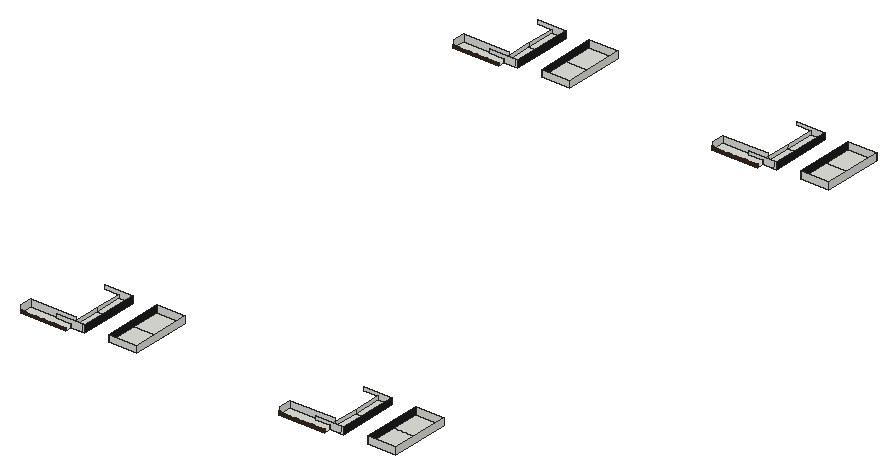
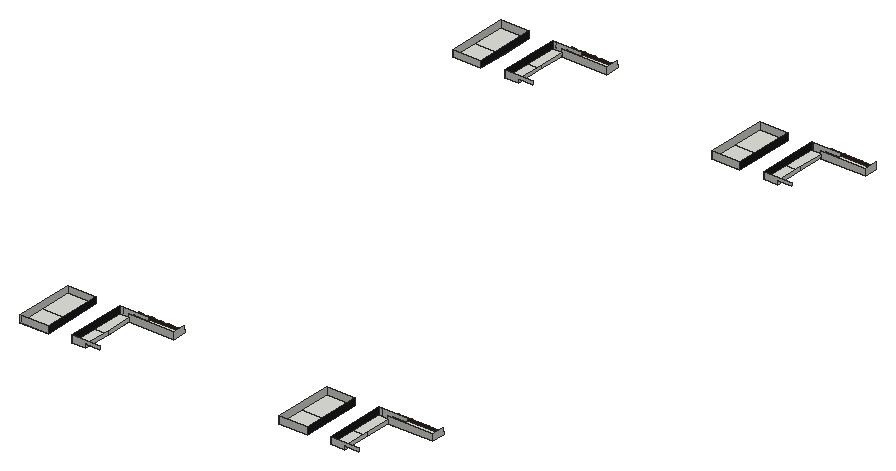
# SketchUp Ruby script. Lengths in inches.
U = 1.inch
M = Sketchup.active_model
def pt(a) = Geom::Point3d.new(a.map { |v| v * U })
def face(e, loops, mat)
  f = e.add_face(loops[0].map { |a| pt(a) })
  loops[1..].each { |l| e.add_face(l.map { |a| pt(a) }).erase! }
  f.material = f.back_material = mat if mat
  f
end
# faces: each face lists its corners as indices into pts; further lists are holes
def faces(e, pts, list, mat = nil) = list.each { |f| face(e, (f[0].is_a?(Array) ? f : [f]).map { |l| l.map { |i| pts[i] } }, mat) }
# xy, xz, yz: faces in a plane at the given z, y or x. An outline is a flat list of corners, or four numbers for a rectangle; further outlines are holes
def ring(l) = l.size == 4 ? [[l[0], l[1]], [l[2], l[1]], [l[2], l[3]], [l[0], l[3]]] : l.each_slice(2).to_a
def flat(e, list, mat, &to3) = list.each { |f| face(e, (f[0].is_a?(Array) ? f : [f]).map { |l| ring(l).map { |u, v| to3.(u, v) } }, mat) }
def xy(e, z, list, mat = nil) = flat(e, list, mat) { |x, y| [x, y, z] }
def xz(e, y, list, mat = nil) = flat(e, list, mat) { |x, z| [x, y, z] }
def yz(e, x, list, mat = nil) = flat(e, list, mat) { |y, z| [x, y, z] }
def lines(e, pts, list) = list.each { |a, b| e.add_line(pt(pts[a]), pt(pts[b])) }
# prism: a flat outline (further loops are holes) pulled along v
def prism(e, loops, v, mat = nil)
  f = face(e, loops, mat); d = Geom::Vector3d.new(v.map { |x| x * U })
  f.pushpull(f.normal.samedirection?(d) ? d.length : -d.length)
end
def box(e, o, s, mat = nil) = prism(e, [[o, [o[0] + s[0], o[1], o[2]], [o[0] + s[0], o[1] + s[1], o[2]], [o[0], o[1] + s[1], o[2]]]], [0, 0, s[2]], mat)
def at(x, y, z, deg = 0) = Geom::Transformation.translation(pt([x, y, z])) * Geom::Transformation.rotation(ORIGIN, Z_AXIS, deg.degrees)
def axes(o, x, y, z) = Geom::Transformation.new([*x, 0, *y, 0, *z, 0, *pt(o).to_a, 1])
def part(name) = M.definitions.add(name)
# library, detail: a bought-in or finely detailed component or shape, given as its bounding box
def library(name, o, s) = part(name).tap { |d| box(d.entities, o, s) }
def detail(e, o, s) = box(e.add_group.entities, o, s)
def put(e, d, t, mat = nil) = e.add_instance(d, t).tap { |i| i.material = mat if mat }
def group(e, t, mat = nil) = e.add_group.tap { |g| g.transformation = t; g.material = mat if mat }.entities
root = M.entities
M.materials.add("[Color M08]").color = [30, 30, 30]
M.materials.add("[Wood Veneer 01]").color = [66, 38, 20]
xy(root,230.89,[[2010.28,566.68,2164.35,611.02],[2889.03,566.68,3043.1,611.02],[2010.28,2402.3,2164.35,2446.65],[2889.03,2402.3,3043.1,2446.65]])
xy(root,231,[[2164.35,589.83,2211.2,697.21],[2291.96,589.83,2387.27,697.21],[3043.1,589.83,3089.95,697.21],[3170.71,589.83,3266.02,697.21],[2164.35,697.21,2211.2,792.52],
  [2291.96,697.21,2387.27,792.52],[3043.1,697.21,3089.95,792.52],[3170.71,697.21,3266.02,792.52],[2164.35,2425.46,2211.2,2532.83],[2291.96,2425.46,2387.27,2532.83],
  [3043.1,2425.46,3089.95,2532.83],[3170.71,2425.46,3266.02,2532.83],[2164.35,2532.83,2211.2,2628.15],[2291.96,2532.83,2387.27,2628.15],[3043.1,2532.83,3089.95,2628.15],
  [3170.71,2532.83,3266.02,2628.15]])
xz(root,566.68,[[2010.28,230.89,2164.35,230.89,2164.35,240.89,2162.52,240.1,2161.96,239.96,2161.4375,239.81,2160.75,239.53,2160.2,239.49,2159.48,239.42,2158.68,239.28,2157.91,239.15,2157.28,238.9,2155.89,238.9,2155.13,238.89,2154.45,238.89,2153.77,238.88,2153.23,238.875,2152.47,238.86,2151.73,238.83,2151.16,238.8,2150.58,238.74,2149.92,238.6,2149.35,238.51,2148.82,238.33,2148.13,238.08,2147.45,237.84,2146.76,237.5625,2146.16,237.47,2145.48,237.4,2144.75,237.42,2144.18,237.45,2143.59,237.51,2142.99,237.59,2142.45,237.71,2141.62,238,2140.91,238.33,2140.36,238.57,2139.86,238.86,2139.34,238.96,2138.65,239.02,2137.97,239.125,2137.23,239.04,2136.66,238.66,2136.07,238.61,2135.41,238.55,2134.89,238.27,2134.21,238.18,2133.53,238.18,2132.86,238.11,2132.33,238.15,2131.51,238.19,2130.9375,238.26,2130.37,238.48,2129.71,238.56,2129.14,238.67,2128.62,239.01,2127.9375,239.18,2127.3125,239.5,2126.55,239.65,2125.9375,239.8,2125.18,239.96,2124.53,240.23,2123.95,240.27,2123.3,240.43,2122.73,240.43,2122.15,240.42,2121.625,240.41,2120.93,240.4,2120.24,240.37,2119.55,240.33,2118.87,240.27,2118.19,240.17,2117.57,239.97,2116.92,239.75,2116.18,239.375,2115.39,239.08,2114.51,238.72,2113.76,238.46,2112.54,238.14,2111.42,237.88,2110.77,237.87,2109.9,237.74,2109.19,237.79,2108.42,237.86,2107.79,238.15,2107.02,238.19,2106.4,238.25,2105.64,238.45,2104.95,238.62,2100.06,238.62,2099.5,238.625,2098.64,238.625,2097.95,238.63,2097.33,238.64,2096.55,238.65,2095.88,238.66,2095.19,238.6875,2094.52,238.73,2094.04,238.78,2093.16,238.93,2092.39,239.07,2091.84,239.16,2090.99,239.44,2090.32,239.56,2089.71,239.72,2088.98,239.7,2088.42,239.69,2087.83,239.65,2087.21,239.6,2086.72,239.54,2085.91,239.31,2084.91,239.22,2084.33,239.12,2083.6875,238.76,2083.05,238.51,2082.49,238.375,2082.05,238.02,2081.35,237.74,2080.73,237.43,2079.88,237.22,2079.2,236.98,2078.59,237.01,2077.9,237.04,2077.14,237.11,2076.45,237.2,2075.92,237.33,2075.25,237.68,2074.3125,237.96,2073.75,238.28,2072.97,238.43,2072.19,238.78,2071.52,238.79,2070.98,238.8,2070.22,238.83,2069.47,238.875,2068.9,238.94,2068.32,239.04,2067.66,239.29,2067.08,239.53,2066.55,239.7,2065.86,239.92,2065.23,240.11,2064.45,240.27,2063.83,240.25,2063.125,240.23,2062.36,240.19,2061.6875,240.12,2061.03,240.03,2060.39,239.85,2059.84,239.52,2059.28,239.35,2058.69,239.18,2058.18,238.86,2057.49,238.72,2056.67,238.59,2056.16,238.34,2050.59,238.34,2049.91,238.33,2048.68,238.33,2047.96,238.32,2047.11,238.3,2046.48,238.28,2045.73,238.26,2045.1,238.15,2044.34,238.13,2043.79,238.1,2042.9375,237.98,2042.32,237.94,2041.56,237.89,2040.89,237.65,2039.58,237.65,2038.89,237.66,2038.14,237.67,2037.54,237.68,2036.93,237.71,2036.22,237.76,2035.53,237.82,2034.87,237.9,2033.93,238.21,2033.46,238.31,2032.55,238.43,2031.9,238.74,2031.32,239.11,2030.74,239.38,2030.28,239.71,2029.58,240.11,2028.89,240.09,2028.23,240.05,2027.64,239.99,2026.91,239.88,2026.36,239.69,2025.78,239.55,2025.22,238.9375,2024.69,238.77,2023.95,238.79,2023.08,238.8,2022.57,238.82,2021.53,238.92,2020.84,238.93,2020.14,238.94,2019.44,238.97,2018.76,239.03,2018.07,239.09,2017.29,239.19,2016.78,239.52,2016.22,239.64,2015.77,239.86,2014.98,240.2,2014.38,240.59,2013.84,240.85,2012.82,241.55,2011.55,241.69,2010.34,241.52,2010.28,241.52],[2889.03,230.89,3043.1,230.89,3043.1,240.89,3041.27,240.1,3040.71,239.96,3040.1875,239.81,3039.5,239.53,3038.95,239.49,3038.23,239.42,3037.43,239.28,3036.66,239.15,3036.03,238.9,3034.64,238.9,3033.88,238.89,3033.2,238.89,3032.52,238.88,3031.98,238.875,3031.22,238.86,3030.48,238.83,3029.91,238.8,3029.33,238.74,3028.67,238.6,3028.1,238.51,3027.57,238.33,3026.88,238.08,3026.2,237.84,3025.51,237.5625,3024.91,237.47,3024.23,237.4,3023.5,237.42,3022.93,237.45,3022.34,237.51,3021.74,237.59,3021.2,237.71,3020.37,238,3019.66,238.33,3019.11,238.57,3018.61,238.86,3018.09,238.96,3017.4,239.02,3016.72,239.125,3015.98,239.04,3015.41,238.66,3014.82,238.61,3014.16,238.55,3013.64,238.27,3012.96,238.18,3012.28,238.18,3011.61,238.11,3011.08,238.15,3010.26,238.19,3009.6875,238.26,3009.12,238.48,3008.46,238.56,3007.89,238.67,3007.37,239.01,3006.6875,239.18,3006.0625,239.5,3005.3,239.65,3004.6875,239.8,3003.93,239.96,3003.28,240.23,3002.7,240.27,3002.05,240.43,3001.48,240.43,3000.9,240.42,3000.375,240.41,2999.68,240.4,2998.99,240.37,2998.3,240.33,2997.62,240.27,2996.94,240.17,2996.32,239.97,2995.67,239.75,2994.93,239.375,2994.14,239.08,2993.26,238.72,2992.51,238.46,2991.29,238.14,2990.17,237.88,2989.52,237.87,2988.65,237.74,2987.94,237.79,2987.17,237.86,2986.54,238.15,2985.77,238.19,2985.15,238.25,2984.39,238.45,2983.7,238.62,2978.81,238.62,2978.25,238.625,2977.39,238.625,2976.7,238.63,2976.08,238.64,2975.3,238.65,2974.63,238.66,2973.94,238.6875,2973.27,238.73,2972.79,238.78,2971.91,238.93,2971.14,239.07,2970.59,239.16,2969.74,239.44,2969.07,239.56,2968.46,239.72,2967.73,239.7,2967.17,239.69,2966.58,239.65,2965.96,239.6,2965.47,239.54,2964.66,239.31,2963.66,239.22,2963.08,239.12,2962.4375,238.76,2961.8,238.51,2961.24,238.375,2960.8,238.02,2960.1,237.74,2959.48,237.43,2958.63,237.22,2957.95,236.98,2957.34,237.01,2956.65,237.04,2955.89,237.11,2955.2,237.2,2954.67,237.33,2954,237.68,2953.0625,237.96,2952.5,238.28,2951.72,238.43,2950.94,238.78,2950.27,238.79,2949.73,238.8,2948.97,238.83,2948.22,238.875,2947.65,238.94,2947.07,239.04,2946.41,239.29,2945.83,239.53,2945.3,239.7,2944.61,239.92,2943.98,240.11,2943.2,240.27,2942.58,240.25,2941.875,240.23,2941.11,240.19,2940.4375,240.12,2939.78,240.03,2939.14,239.85,2938.59,239.52,2938.03,239.35,2937.44,239.18,2936.93,238.86,2936.24,238.72,2935.42,238.59,2934.91,238.34,2929.34,238.34,2928.66,238.33,2927.43,238.33,2926.71,238.32,2925.86,238.3,2925.23,238.28,2924.48,238.26,2923.85,238.15,2923.09,238.13,2922.54,238.1,2921.6875,237.98,2921.07,237.94,2920.31,237.89,2919.64,237.65,2918.33,237.65,2917.64,237.66,2916.89,237.67,2916.29,237.68,2915.68,237.71,2914.97,237.76,2914.28,237.82,2913.62,237.9,2912.68,238.21,2912.21,238.31,2911.3,238.43,2910.65,238.74,2910.07,239.11,2909.49,239.38,2909.03,239.71,2908.33,240.11,2907.64,240.09,2906.98,240.05,2906.39,239.99,2905.66,239.88,2905.11,239.69,2904.53,239.55,2903.97,238.9375,2903.44,238.77,2902.7,238.79,2901.83,238.8,2901.32,238.82,2900.28,238.92,2899.59,238.93,2898.89,238.94,2898.19,238.97,2897.51,239.03,2896.82,239.09,2896.04,239.19,2895.53,239.52,2894.97,239.64,2894.52,239.86,2893.73,240.2,2893.13,240.59,2892.59,240.85,2891.57,241.55,2890.3,241.69,2889.09,241.52,2889.03,241.52]],"[Wood Veneer 01]")
xz(root,589.83,[[2164.35,231,2202.28,231,2202.28,254.5,2115.89,254.5,2115.89,242.625,2164.35,242.625],[2202.28,231,2211.2,254.5],[2291.96,231,2387.27,254.5],[3043.1,231,3081.03,231,3081.03,254.5,2994.64,254.5,2994.64,242.625,3043.1,242.625],[3081.03,231,3089.95,254.5],
  [3170.71,231,3266.02,254.5]])
xz(root,611.02,[[2010.28,230.89,2164.35,254.5],[2889.03,230.89,3043.1,254.5]])
xz(root,792.52,[[2164.35,231,2164.35,242.625,2115.89,242.625,2115.89,254.5,2211.2,254.5,2211.2,231],[2291.96,231,2387.27,254.5],[3043.1,231,3043.1,242.625,2994.64,242.625,2994.64,254.5,3089.95,254.5,3089.95,231],[3170.71,231,3266.02,254.5]])
xz(root,2402.3,[[2010.28,230.89,2164.35,230.89,2164.35,240.89,2162.52,240.1,2161.96,239.96,2161.4375,239.81,2160.75,239.53,2160.2,239.49,2159.48,239.42,2158.68,239.28,2157.91,239.15,2157.28,238.9,2155.89,238.9,2155.13,238.89,2154.45,238.89,2153.77,238.88,2153.23,238.875,2152.47,238.86,2151.73,238.83,2151.16,238.8,2150.58,238.74,2149.92,238.6,2149.35,238.51,2148.82,238.33,2148.13,238.08,2147.45,237.84,2146.76,237.5625,2146.16,237.47,2145.48,237.4,2144.75,237.42,2144.18,237.45,2143.59,237.51,2142.99,237.59,2142.45,237.71,2141.62,238,2140.91,238.33,2140.36,238.57,2139.86,238.86,2139.34,238.96,2138.65,239.02,2137.97,239.125,2137.23,239.04,2136.66,238.66,2136.07,238.61,2135.41,238.55,2134.89,238.27,2134.21,238.18,2133.53,238.18,2132.86,238.11,2132.33,238.15,2131.51,238.19,2130.9375,238.26,2130.37,238.48,2129.71,238.56,2129.14,238.67,2128.62,239.01,2127.9375,239.18,2127.3125,239.5,2126.55,239.65,2125.9375,239.8,2125.18,239.96,2124.53,240.23,2123.95,240.27,2123.3,240.43,2122.73,240.43,2122.15,240.42,2121.625,240.41,2120.93,240.4,2120.24,240.37,2119.55,240.33,2118.87,240.27,2118.19,240.17,2117.57,239.97,2116.92,239.75,2116.18,239.375,2115.39,239.08,2114.51,238.72,2113.76,238.46,2112.54,238.14,2111.42,237.88,2110.77,237.87,2109.9,237.74,2109.19,237.79,2108.42,237.86,2107.79,238.15,2107.02,238.19,2106.4,238.25,2105.64,238.45,2104.95,238.62,2100.06,238.62,2099.5,238.625,2098.64,238.625,2097.95,238.63,2097.33,238.64,2096.55,238.65,2095.88,238.66,2095.19,238.6875,2094.52,238.73,2094.04,238.78,2093.16,238.93,2092.39,239.07,2091.84,239.16,2090.99,239.44,2090.32,239.56,2089.71,239.72,2088.98,239.7,2088.42,239.69,2087.83,239.65,2087.21,239.6,2086.72,239.54,2085.91,239.31,2084.91,239.22,2084.33,239.12,2083.6875,238.76,2083.05,238.51,2082.49,238.375,2082.05,238.02,2081.35,237.74,2080.73,237.43,2079.88,237.22,2079.2,236.98,2078.59,237.01,2077.9,237.04,2077.14,237.11,2076.45,237.2,2075.92,237.33,2075.25,237.68,2074.3125,237.96,2073.75,238.28,2072.97,238.43,2072.19,238.78,2071.52,238.79,2070.98,238.8,2070.22,238.83,2069.47,238.875,2068.9,238.94,2068.32,239.04,2067.66,239.29,2067.08,239.53,2066.55,239.7,2065.86,239.92,2065.23,240.11,2064.45,240.27,2063.83,240.25,2063.125,240.23,2062.36,240.19,2061.6875,240.12,2061.03,240.03,2060.39,239.85,2059.84,239.52,2059.28,239.35,2058.69,239.18,2058.18,238.86,2057.49,238.72,2056.67,238.59,2056.16,238.34,2050.59,238.34,2049.91,238.33,2048.68,238.33,2047.96,238.32,2047.11,238.3,2046.48,238.28,2045.73,238.26,2045.1,238.15,2044.34,238.13,2043.79,238.1,2042.9375,237.98,2042.32,237.94,2041.56,237.89,2040.89,237.65,2039.58,237.65,2038.89,237.66,2038.14,237.67,2037.54,237.68,2036.93,237.71,2036.22,237.76,2035.53,237.82,2034.87,237.9,2033.93,238.21,2033.46,238.31,2032.55,238.43,2031.9,238.74,2031.32,239.11,2030.74,239.38,2030.28,239.71,2029.58,240.11,2028.89,240.09,2028.23,240.05,2027.64,239.99,2026.91,239.88,2026.36,239.69,2025.78,239.55,2025.22,238.9375,2024.69,238.77,2023.95,238.79,2023.08,238.8,2022.57,238.82,2021.53,238.92,2020.84,238.93,2020.14,238.94,2019.44,238.97,2018.76,239.03,2018.07,239.09,2017.29,239.19,2016.78,239.52,2016.22,239.64,2015.77,239.86,2014.98,240.2,2014.38,240.59,2013.84,240.85,2012.82,241.55,2011.55,241.69,2010.34,241.52,2010.28,241.52],[2889.03,230.89,3043.1,230.89,3043.1,240.89,3041.27,240.1,3040.71,239.96,3040.1875,239.81,3039.5,239.53,3038.95,239.49,3038.23,239.42,3037.43,239.28,3036.66,239.15,3036.03,238.9,3034.64,238.9,3033.88,238.89,3033.2,238.89,3032.52,238.88,3031.98,238.875,3031.22,238.86,3030.48,238.83,3029.91,238.8,3029.33,238.74,3028.67,238.6,3028.1,238.51,3027.57,238.33,3026.88,238.08,3026.2,237.84,3025.51,237.5625,3024.91,237.47,3024.23,237.4,3023.5,237.42,3022.93,237.45,3022.34,237.51,3021.74,237.59,3021.2,237.71,3020.37,238,3019.66,238.33,3019.11,238.57,3018.61,238.86,3018.09,238.96,3017.4,239.02,3016.72,239.125,3015.98,239.04,3015.41,238.66,3014.82,238.61,3014.16,238.55,3013.64,238.27,3012.96,238.18,3012.28,238.18,3011.61,238.11,3011.08,238.15,3010.26,238.19,3009.6875,238.26,3009.12,238.48,3008.46,238.56,3007.89,238.67,3007.37,239.01,3006.6875,239.18,3006.0625,239.5,3005.3,239.65,3004.6875,239.8,3003.93,239.96,3003.28,240.23,3002.7,240.27,3002.05,240.43,3001.48,240.43,3000.9,240.42,3000.375,240.41,2999.68,240.4,2998.99,240.37,2998.3,240.33,2997.62,240.27,2996.94,240.17,2996.32,239.97,2995.67,239.75,2994.93,239.375,2994.14,239.08,2993.26,238.72,2992.51,238.46,2991.29,238.14,2990.17,237.88,2989.52,237.87,2988.65,237.74,2987.94,237.79,2987.17,237.86,2986.54,238.15,2985.77,238.19,2985.15,238.25,2984.39,238.45,2983.7,238.62,2978.81,238.62,2978.25,238.625,2977.39,238.625,2976.7,238.63,2976.08,238.64,2975.3,238.65,2974.63,238.66,2973.94,238.6875,2973.27,238.73,2972.79,238.78,2971.91,238.93,2971.14,239.07,2970.59,239.16,2969.74,239.44,2969.07,239.56,2968.46,239.72,2967.73,239.7,2967.17,239.69,2966.58,239.65,2965.96,239.6,2965.47,239.54,2964.66,239.31,2963.66,239.22,2963.08,239.12,2962.4375,238.76,2961.8,238.51,2961.24,238.375,2960.8,238.02,2960.1,237.74,2959.48,237.43,2958.63,237.22,2957.95,236.98,2957.34,237.01,2956.65,237.04,2955.89,237.11,2955.2,237.2,2954.67,237.33,2954,237.68,2953.0625,237.96,2952.5,238.28,2951.72,238.43,2950.94,238.78,2950.27,238.79,2949.73,238.8,2948.97,238.83,2948.22,238.875,2947.65,238.94,2947.07,239.04,2946.41,239.29,2945.83,239.53,2945.3,239.7,2944.61,239.92,2943.98,240.11,2943.2,240.27,2942.58,240.25,2941.875,240.23,2941.11,240.19,2940.4375,240.12,2939.78,240.03,2939.14,239.85,2938.59,239.52,2938.03,239.35,2937.44,239.18,2936.93,238.86,2936.24,238.72,2935.42,238.59,2934.91,238.34,2929.34,238.34,2928.66,238.33,2927.43,238.33,2926.71,238.32,2925.86,238.3,2925.23,238.28,2924.48,238.26,2923.85,238.15,2923.09,238.13,2922.54,238.1,2921.6875,237.98,2921.07,237.94,2920.31,237.89,2919.64,237.65,2918.33,237.65,2917.64,237.66,2916.89,237.67,2916.29,237.68,2915.68,237.71,2914.97,237.76,2914.28,237.82,2913.62,237.9,2912.68,238.21,2912.21,238.31,2911.3,238.43,2910.65,238.74,2910.07,239.11,2909.49,239.38,2909.03,239.71,2908.33,240.11,2907.64,240.09,2906.98,240.05,2906.39,239.99,2905.66,239.88,2905.11,239.69,2904.53,239.55,2903.97,238.9375,2903.44,238.77,2902.7,238.79,2901.83,238.8,2901.32,238.82,2900.28,238.92,2899.59,238.93,2898.89,238.94,2898.19,238.97,2897.51,239.03,2896.82,239.09,2896.04,239.19,2895.53,239.52,2894.97,239.64,2894.52,239.86,2893.73,240.2,2893.13,240.59,2892.59,240.85,2891.57,241.55,2890.3,241.69,2889.09,241.52,2889.03,241.52]],"[Wood Veneer 01]")
xz(root,2425.46,[[2164.35,231,2202.28,231,2202.28,254.5,2115.89,254.5,2115.89,242.625,2164.35,242.625],[2202.28,231,2211.2,254.5],[2291.96,231,2387.27,254.5],[3043.1,231,3081.03,231,3081.03,254.5,2994.64,254.5,2994.64,242.625,3043.1,242.625],[3081.03,231,3089.95,254.5],
  [3170.71,231,3266.02,254.5]])
xz(root,2446.65,[[2010.28,230.89,2164.35,254.5],[2889.03,230.89,3043.1,254.5]])
xz(root,2628.15,[[2164.35,231,2164.35,242.625,2115.89,242.625,2115.89,254.5,2211.2,254.5,2211.2,231],[2291.96,231,2387.27,254.5],[3043.1,231,3043.1,242.625,2994.64,242.625,2994.64,254.5,3089.95,254.5,3089.95,231],[3170.71,231,3266.02,254.5]])
yz(root,2010.28,[[566.68,230.89,566.68,241.52,568.68,241.52,568.68,254.5,611.02,254.5,611.02,230.89],[2402.3,230.89,2402.3,241.52,2404.3,241.52,2404.3,254.5,2446.65,254.5,2446.65,230.89]])
yz(root,2164.35,[[589.83,230.89,611.02,231],[2425.46,230.89,2446.65,231],[589.83,231,611.02,242.625],[611.02,231,697.21,242.625],[697.21,231,792.52,242.625],
  [2425.46,231,2446.65,242.625],[2446.65,231,2532.83,242.625],[2532.83,231,2628.15,242.625]])
yz(root,2211.2,[[589.83,231,792.52,254.5],[2425.46,231,2628.15,254.5]],"[Color M08]")
yz(root,2291.96,[[589.83,231,792.52,254.5],[2425.46,231,2628.15,254.5]],"[Color M08]")
yz(root,2387.27,[[589.83,231,792.52,254.5],[2425.46,231,2628.15,254.5]])
yz(root,2889.03,[[566.68,230.89,566.68,241.52,568.68,241.52,568.68,254.5,611.02,254.5,611.02,230.89],[2402.3,230.89,2402.3,241.52,2404.3,241.52,2404.3,254.5,2446.65,254.5,2446.65,230.89]])
yz(root,3043.1,[[589.83,230.89,611.02,231],[2425.46,230.89,2446.65,231],[589.83,231,611.02,242.625],[611.02,231,697.21,242.625],[697.21,231,792.52,242.625],
  [2425.46,231,2446.65,242.625],[2446.65,231,2532.83,242.625],[2532.83,231,2628.15,242.625]])
yz(root,3089.95,[[589.83,231,792.52,254.5],[2425.46,231,2628.15,254.5]],"[Color M08]")
yz(root,3170.71,[[589.83,231,792.52,254.5],[2425.46,231,2628.15,254.5]],"[Color M08]")
yz(root,3266.02,[[589.83,231,792.52,254.5],[2425.46,231,2628.15,254.5]])
